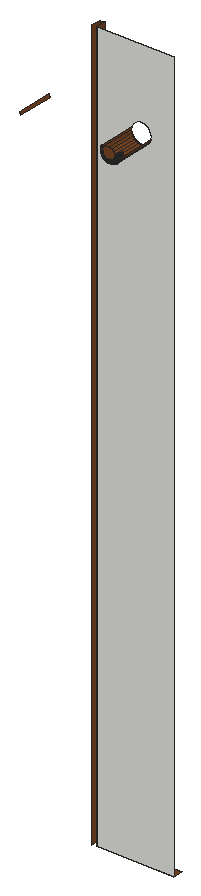
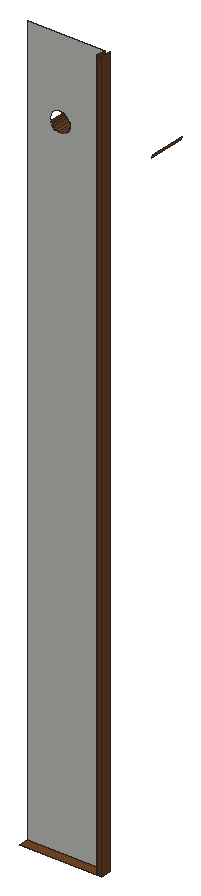
# SketchUp Ruby script. Lengths in inches.
U = 1.inch
M = Sketchup.active_model
def pt(a) = Geom::Point3d.new(a.map { |v| v * U })
def face(e, loops, mat)
  f = e.add_face(loops[0].map { |a| pt(a) })
  loops[1..].each { |l| e.add_face(l.map { |a| pt(a) }).erase! }
  f.material = f.back_material = mat if mat
  f
end
# faces: each face lists its corners as indices into pts; further lists are holes
def faces(e, pts, list, mat = nil) = list.each { |f| face(e, (f[0].is_a?(Array) ? f : [f]).map { |l| l.map { |i| pts[i] } }, mat) }
# xy, xz, yz: faces in a plane at the given z, y or x. An outline is a flat list of corners, or four numbers for a rectangle; further outlines are holes
def ring(l) = l.size == 4 ? [[l[0], l[1]], [l[2], l[1]], [l[2], l[3]], [l[0], l[3]]] : l.each_slice(2).to_a
def flat(e, list, mat, &to3) = list.each { |f| face(e, (f[0].is_a?(Array) ? f : [f]).map { |l| ring(l).map { |u, v| to3.(u, v) } }, mat) }
def xy(e, z, list, mat = nil) = flat(e, list, mat) { |x, y| [x, y, z] }
def xz(e, y, list, mat = nil) = flat(e, list, mat) { |x, z| [x, y, z] }
def yz(e, x, list, mat = nil) = flat(e, list, mat) { |y, z| [x, y, z] }
def lines(e, pts, list) = list.each { |a, b| e.add_line(pt(pts[a]), pt(pts[b])) }
# prism: a flat outline (further loops are holes) pulled along v
def prism(e, loops, v, mat = nil)
  f = face(e, loops, mat); d = Geom::Vector3d.new(v.map { |x| x * U })
  f.pushpull(f.normal.samedirection?(d) ? d.length : -d.length)
end
def box(e, o, s, mat = nil) = prism(e, [[o, [o[0] + s[0], o[1], o[2]], [o[0] + s[0], o[1] + s[1], o[2]], [o[0], o[1] + s[1], o[2]]]], [0, 0, s[2]], mat)
def at(x, y, z, deg = 0) = Geom::Transformation.translation(pt([x, y, z])) * Geom::Transformation.rotation(ORIGIN, Z_AXIS, deg.degrees)
def axes(o, x, y, z) = Geom::Transformation.new([*x, 0, *y, 0, *z, 0, *pt(o).to_a, 1])
def part(name) = M.definitions.add(name)
# library, detail: a bought-in or finely detailed component or shape, given as its bounding box
def library(name, o, s) = part(name).tap { |d| box(d.entities, o, s) }
def detail(e, o, s) = box(e.add_group.entities, o, s)
def put(e, d, t, mat = nil) = e.add_instance(d, t).tap { |i| i.material = mat if mat }
def group(e, t, mat = nil) = e.add_group.tap { |g| g.transformation = t; g.material = mat if mat }.entities
root = M.entities
M.materials.add("[Wood Veneer 01]").color = [120, 70, 37]
xy(root,1.59,[[30.5,2,34.26,2.47]],"[Wood Veneer 01]")
xz(root,0,[[32.68,33.35,32.68,33.36,32.6,33.375,32.59,33.36],[32.68,33.35,32.77,33.36,32.76,33.375,32.68,33.36],[32.59,33.36,32.6,33.375,32.52,33.41,32.51,33.39],[32.68,33.36,32.68,33.38,32.6,33.39,32.6,33.375],[32.68,33.36,32.76,33.375,32.76,33.39,32.68,33.38],
  [32.77,33.36,32.85,33.39,32.84,33.41,32.76,33.375],[32.6,33.375,32.6,33.39,32.53,33.42,32.52,33.41],[32.76,33.375,32.84,33.41,32.83,33.42,32.76,33.39],[32.68,33.38,32.68,33.4,32.61,33.41,32.6,33.39],[32.68,33.38,32.76,33.39,32.75,33.41,32.68,33.4],
  [32.51,33.39,32.52,33.41,32.45,33.46,32.44,33.45],[32.6,33.39,32.61,33.41,32.54,33.4375,32.53,33.42],[32.76,33.39,32.83,33.42,32.82,33.4375,32.75,33.41],[32.85,33.39,32.92,33.45,32.9,33.46,32.84,33.41],[32.68,33.4,32.75,33.41,32.82,33.4375,32.88,33.48,32.93,33.54,32.95,33.61,32.96,33.68,32.95,33.76,32.93,33.83,32.88,33.88,32.82,33.93,32.75,33.96,32.68,33.97,32.61,33.96,32.54,33.93,32.48,33.88,32.43,33.83,32.4,33.76,32.39,33.68,32.4,33.61,32.43,33.54,32.48,33.48,32.54,33.4375,32.61,33.41],
  [32.52,33.41,32.53,33.42,32.47,33.47,32.45,33.46],[32.84,33.41,32.9,33.46,32.89,33.47,32.83,33.42],[32.53,33.42,32.54,33.4375,32.48,33.48,32.47,33.47],[32.83,33.42,32.89,33.47,32.88,33.48,32.82,33.4375],[32.44,33.45,32.45,33.46,32.4,33.52,32.39,33.52],
  [32.92,33.45,32.97,33.52,32.96,33.52,32.9,33.46],[32.45,33.46,32.47,33.47,32.42,33.53,32.4,33.52],[32.9,33.46,32.96,33.52,32.94,33.53,32.89,33.47],[32.47,33.47,32.48,33.48,32.43,33.54,32.42,33.53],[32.89,33.47,32.94,33.53,32.93,33.54,32.88,33.48],
  [32.39,33.52,32.4,33.52,32.37,33.6,32.36,33.6],[32.4,33.52,32.42,33.53,32.39,33.61,32.37,33.6],[32.96,33.52,32.99,33.6,32.97,33.61,32.94,33.53],[32.96,33.52,32.97,33.52,33,33.6,32.99,33.6],[32.42,33.53,32.43,33.54,32.4,33.61,32.39,33.61],
  [32.94,33.53,32.97,33.61,32.95,33.61,32.93,33.54],[32.36,33.6,32.37,33.6,32.36,33.68,32.34,33.68],[32.37,33.6,32.39,33.61,32.38,33.68,32.36,33.68],[32.99,33.6,33,33.68,32.98,33.68,32.97,33.61],[32.99,33.6,33,33.6,33.01,33.68,33,33.68],
  [32.39,33.61,32.4,33.61,32.39,33.68,32.38,33.68],[32.95,33.61,32.97,33.61,32.98,33.68,32.96,33.68],[32.34,33.68,32.36,33.68,32.37,33.77,32.36,33.77],[32.36,33.68,32.38,33.68,32.39,33.76,32.37,33.77],[32.38,33.68,32.39,33.68,32.4,33.76,32.39,33.76],
  [32.96,33.68,32.98,33.68,32.97,33.76,32.95,33.76],[32.98,33.68,33,33.68,32.99,33.77,32.97,33.76],[33,33.68,33.01,33.68,33,33.77,32.99,33.77]],"[Wood Veneer 01]")
xz(root,0.01,[[32.68,33.3,32.68,33.32,32.58,33.33,32.58,33.32],[32.68,33.3,32.78,33.32,32.77,33.33,32.68,33.32],[32.58,33.32,32.58,33.33,32.5,33.37,32.49,33.36],[32.68,33.32,32.68,33.33,32.59,33.34,32.58,33.33],[32.68,33.32,32.77,33.33,32.77,33.34,32.68,33.33],
  [32.78,33.32,32.87,33.36,32.86,33.37,32.77,33.33],[32.58,33.33,32.59,33.34,32.5,33.38,32.5,33.37],[32.77,33.33,32.86,33.37,32.85,33.38,32.77,33.34],[32.49,33.36,32.5,33.37,32.42,33.43,32.41,33.42],[32.87,33.36,32.95,33.42,32.9375,33.43,32.86,33.37],
  [32.5,33.37,32.5,33.38,32.43,33.44,32.42,33.43],[32.86,33.37,32.9375,33.43,32.93,33.44,32.85,33.38],[32.41,33.42,32.42,33.43,32.36,33.5,32.35,33.49],[32.95,33.42,33.01,33.49,33,33.5,32.9375,33.43],[32.42,33.43,32.43,33.44,32.375,33.51,32.36,33.5],
  [32.9375,33.43,33,33.5,32.98,33.51,32.93,33.44],[32.35,33.49,32.36,33.5,32.33,33.59,32.3125,33.59],[33.01,33.49,33.05,33.59,33.03,33.59,33,33.5],[32.36,33.5,32.375,33.51,32.34,33.59,32.33,33.59],[33,33.5,33.03,33.59,33.02,33.59,32.98,33.51],
  [32.3125,33.59,32.33,33.59,32.3125,33.68,32.3,33.68],[32.33,33.59,32.34,33.59,32.33,33.68,32.3125,33.68],[33.02,33.59,33.03,33.59,33.04,33.68,33.03,33.68],[33.03,33.59,33.05,33.59,33.06,33.68,33.04,33.68],[32.3,33.68,32.3125,33.68,32.33,33.78,32.3125,33.78],
  [32.3125,33.68,32.33,33.68,32.34,33.77,32.33,33.78],[33.03,33.68,33.04,33.68,33.03,33.78,33.02,33.77],[33.04,33.68,33.06,33.68,33.05,33.78,33.03,33.78]],"[Wood Veneer 01]")
xz(root,0.02,[[32.68,33.28,32.68,33.29,32.58,33.3,32.57,33.29],[32.68,33.28,32.78,33.29,32.78,33.3,32.68,33.29],[32.57,33.29,32.58,33.3,32.48,33.34,32.48,33.33],[32.78,33.29,32.88,33.33,32.875,33.34,32.78,33.3],[32.48,33.33,32.48,33.34,32.4,33.41,32.39,33.4],
  [32.88,33.33,32.97,33.4,32.96,33.41,32.875,33.34],[32.39,33.4,32.4,33.41,32.34,33.49,32.33,33.48],[32.97,33.4,33.03,33.48,33.02,33.49,32.96,33.41],[32.33,33.48,32.34,33.49,32.3,33.58,32.29,33.58],[33.03,33.48,33.07,33.58,33.06,33.58,33.02,33.49],
  [32.29,33.58,32.3,33.58,32.29,33.68,32.28,33.68],[33.06,33.58,33.07,33.58,33.08,33.68,33.07,33.68],[32.28,33.68,32.29,33.68,32.3,33.78,32.29,33.79],[33.07,33.68,33.08,33.68,33.07,33.79,33.06,33.78]],"[Wood Veneer 01]")
xz(root,0.04,[[32.68,33.25,32.68,33.26,32.57,33.27,32.57,33.26],[32.68,33.25,32.79,33.26,32.79,33.27,32.68,33.26],[32.57,33.26,32.57,33.27,32.47,33.3125,32.46,33.31],[32.79,33.26,32.9,33.31,32.89,33.3125,32.79,33.27],[32.46,33.31,32.47,33.3125,32.38,33.38,32.37,33.375],
  [32.9,33.31,32.99,33.375,32.98,33.38,32.89,33.3125],[32.37,33.375,32.38,33.38,32.31,33.47,32.3,33.46],[32.99,33.375,33.06,33.46,33.05,33.47,32.98,33.38],[32.3,33.46,32.31,33.47,32.27,33.57,32.26,33.57],[33.06,33.46,33.1,33.57,33.09,33.57,33.05,33.47],
  [32.26,33.57,32.27,33.57,32.25,33.68,32.24,33.68],[33.09,33.57,33.1,33.57,33.12,33.68,33.11,33.68],[32.24,33.68,32.25,33.68,32.27,33.79,32.26,33.8],[33.11,33.68,33.12,33.68,33.1,33.8,33.09,33.79]],"[Wood Veneer 01]")
xz(root,2,[[[30.5,1.59,34.26,37.59],[32.68,33.18,32.55,33.2,32.43,33.25,32.33,33.33,32.25,33.43,32.2,33.55,32.18,33.68,32.2,33.8125,32.25,33.93,32.33,34.04,32.43,34.12,32.55,34.17,32.68,34.18,32.81,34.17,32.93,34.12,33.03,34.04,33.11,33.93,33.16,33.8125,33.18,33.68,33.16,33.55,33.11,33.43,33.03,33.33,32.93,33.25,32.81,33.2]]])
xz(root,2.47,[[30.26,1.59,30.5,37.59]],"[Wood Veneer 01]")
yz(root,30.26,[[2,1.59,2.47,37.59]],"[Wood Veneer 01]")
yz(root,30.5,[[2,1.59,2.47,37.59]],"[Wood Veneer 01]")
p = [[32.5625,0.05,33.25],[32.68,0.05,33.24],[32.68,0.04,33.25],[32.57,0.04,33.26],[32.79,0.04,33.26],[32.79,0.05,33.25],
  [32.55,0.15,33.21],[32.43,0.15,33.26],[32.43,0.16,33.25],[32.55,0.16,33.2],[32.55,0.13,33.21],[32.43,0.13,33.26],
  [32.55,0.12,33.21],[32.4375,0.12,33.26],[32.55,0.11,33.22],[32.4375,0.11,33.27],[32.56,0.09,33.22],[32.44,0.09,33.27],
  [32.56,0.08,33.23],[32.44,0.08,33.28],[32.56,0.07,33.24],[32.45,0.07,33.28],[32.5625,0.0625,33.24],[32.45,0.0625,33.29],
  [32.46,0.05,33.3],[32.68,0.16,33.1875],[32.68,0.15,33.1875],[32.68,0.13,33.19],[32.68,0.12,33.2],[32.68,0.11,33.2],
  [32.68,0.09,33.21],[32.68,0.08,33.21],[32.68,0.07,33.22],[32.68,0.0625,33.23],[32.8,0.0625,33.24],[32.8,0.07,33.24],
  [32.8,0.08,33.23],[32.8,0.09,33.22],[32.8,0.11,33.22],[32.81,0.12,33.21],[32.81,0.13,33.21],[32.81,0.15,33.21],
  [32.81,0.16,33.2],[32.91,0.0625,33.29],[32.9,0.05,33.3],[32.91,0.07,33.28],[32.91,0.08,33.28],[32.92,0.09,33.27],
  [32.92,0.11,33.27],[32.92,0.12,33.26],[32.92,0.13,33.26],[32.93,0.15,33.26],[32.93,0.16,33.25],[32.43,2,33.25],
  [32.55,2,33.2],[32.55,0.21,33.2],[32.43,0.21,33.25],[32.55,0.2,33.2],[32.43,0.2,33.25],[32.55,0.18,33.2],
  [32.43,0.18,33.25],[32.68,2,33.18],[32.68,0.21,33.18],[32.68,0.2,33.18],[32.68,0.18,33.18],[32.81,0.18,33.2],
  [32.81,0.2,33.2],[32.81,0.21,33.2],[32.81,2,33.2],[32.93,0.18,33.25],[32.93,0.2,33.25],[32.93,0.21,33.25],
  [32.93,2,33.25],[32.36,0.05,33.37],[32.46,0.04,33.31],[32.37,0.04,33.375],[32.38,0.04,33.38],[32.47,0.04,33.3125],
  [32.47,0.03,33.32],[32.39,0.03,33.39],[32.48,0.02,33.33],[32.39,0.02,33.4],[32.4,0.02,33.41],[32.48,0.02,33.34],
  [32.49,0.01,33.36],[32.41,0.01,33.42],[32.57,0.03,33.28],[32.57,0.04,33.27],[32.57,0.02,33.29],[32.58,0.01,33.32],
  [32.58,0.02,33.3],[32.59,0,33.36],[32.51,0,33.39],[32.5,0.01,33.38],[32.59,0.01,33.34],[32.68,0.04,33.26],
  [32.68,0.03,33.27],[32.68,0.02,33.28],[32.68,0.02,33.29],[32.68,0.01,33.3],[32.68,0.01,33.33],[32.68,0,33.35],
  [32.77,0,33.36],[32.77,0.01,33.34],[32.78,0.01,33.32],[32.78,0.02,33.3],[32.78,0.02,33.29],[32.79,0.03,33.28],
  [32.79,0.04,33.27],[32.85,0.01,33.38],[32.85,0,33.39],[32.875,0.02,33.34],[32.87,0.01,33.36],[32.89,0.03,33.32],
  [32.88,0.02,33.33],[32.89,0.04,33.3125],[32.9,0.04,33.31],[32.96,0.02,33.41],[32.95,0.01,33.42],[32.97,0.03,33.39],
  [32.97,0.02,33.4],[32.98,0.04,33.38],[32.99,0.05,33.37],[32.99,0.04,33.375],[32.33,0.15,33.33],[32.25,0.15,33.4375],
  [32.25,0.16,33.43],[32.33,0.16,33.33],[32.33,0.13,33.34],[32.25,0.13,33.4375],[32.34,0.12,33.34],[32.26,0.12,33.44],
  [32.34,0.11,33.34],[32.26,0.11,33.44],[32.34,0.09,33.35],[32.27,0.09,33.45],[32.35,0.08,33.35],[32.27,0.08,33.45],
  [32.35,0.07,33.36],[32.36,0.0625,33.36],[33,0.0625,33.36],[33.01,0.07,33.36],[33.01,0.08,33.35],[33.02,0.09,33.35],
  [33.02,0.11,33.34],[33.02,0.12,33.34],[33.03,0.13,33.34],[33.03,0.15,33.33],[33.03,0.16,33.33],[33.09,0.09,33.45],
  [33.09,0.08,33.45],[33.1,0.11,33.44],[33.1,0.12,33.44],[33.1,0.13,33.4375],[33.11,0.15,33.4375],[33.11,0.16,33.43],
  [32.25,2,33.43],[32.33,2,33.33],[32.33,0.21,33.33],[32.25,0.21,33.43],[32.33,0.2,33.33],[32.25,0.2,33.43],
  [32.33,0.18,33.33],[32.25,0.18,33.43],[33.03,0.18,33.33],[33.03,0.2,33.33],[33.03,0.21,33.33],[33.03,2,33.33],
  [33.11,0.18,33.43],[33.11,0.2,33.43],[33.11,0.21,33.43],[33.11,2,33.43],[32.3,0.04,33.46],[32.29,0.05,33.46],
  [32.32,0.03,33.48],[32.31,0.04,33.47],[32.33,0.02,33.48],[32.35,0.01,33.49],[32.34,0.02,33.49],[32.44,0,33.45],
  [32.39,0,33.52],[32.375,0.01,33.51],[32.43,0.01,33.44],[32.93,0.01,33.44],[32.92,0,33.45],[32.98,0.01,33.51],
  [32.97,0,33.52],[33.02,0.02,33.49],[33.01,0.01,33.49],[33.04,0.03,33.48],[33.03,0.02,33.48],[33.05,0.04,33.47],
  [33.07,0.05,33.46],[33.06,0.04,33.46],[32.2,0.16,33.55],[32.2,0.15,33.56],[32.21,0.13,33.56],[32.21,0.12,33.56],
  [32.21,0.11,33.56],[32.22,0.09,33.56],[32.23,0.08,33.5625],[32.28,0.07,33.45],[32.23,0.07,33.5625],[32.29,0.0625,33.46],
  [33.07,0.0625,33.46],[33.08,0.07,33.45],[33.125,0.07,33.5625],[33.13,0.08,33.5625],[33.14,0.09,33.56],[33.14,0.11,33.56],
  [33.15,0.12,33.56],[33.15,0.13,33.56],[33.16,0.15,33.56],[33.16,0.16,33.55],[32.2,2,33.55],[32.2,0.21,33.55],
  [32.2,0.2,33.55],[32.2,0.18,33.55],[33.16,0.18,33.55],[33.16,0.2,33.55],[33.16,0.21,33.55],[33.16,2,33.55],
  [32.25,0.05,33.57],[32.26,0.04,33.57],[32.27,0.04,33.57],[32.28,0.03,33.58],[32.29,0.02,33.58],[32.3,0.02,33.58],
  [32.3125,0.01,33.59],[32.34,0.01,33.59],[32.36,0,33.6],[33,0,33.6],[33.02,0.01,33.59],[33.05,0.01,33.59],
  [33.06,0.02,33.58],[33.07,0.02,33.58],[33.08,0.03,33.58],[33.09,0.04,33.57],[33.1,0.04,33.57],[33.11,0.05,33.57],
  [32.24,0.0625,33.57],[33.12,0.0625,33.57],[32.23,0.05,33.68],[32.24,0.04,33.68],[32.25,0.04,33.68],[32.26,0.03,33.68],
  [32.28,0.02,33.68],[32.29,0.02,33.68],[32.3,0.01,33.68],[32.33,0.01,33.68],[32.34,0,33.68],[33.01,0,33.68],
  [33.03,0.01,33.68],[33.06,0.01,33.68],[33.07,0.02,33.68],[33.08,0.02,33.68],[33.1,0.03,33.68],[33.11,0.04,33.68],
  [33.12,0.04,33.68],[33.125,0.05,33.68],[32.18,0.16,33.68],[32.19,0.15,33.68],[32.1875,0.13,33.68],[32.19,0.12,33.68],
  [32.2,0.11,33.68],[32.2,0.09,33.68],[32.21,0.08,33.68],[32.22,0.07,33.68],[32.22,0.0625,33.68],[33.13,0.0625,33.68],
  [33.14,0.07,33.68],[33.15,0.08,33.68],[33.16,0.09,33.68],[33.16,0.11,33.68],[33.17,0.12,33.68],[33.17,0.13,33.68],
  [33.17,0.15,33.68],[33.18,0.16,33.68],[32.18,2,33.68],[32.18,0.21,33.68],[32.18,0.2,33.68],[32.18,0.18,33.68],
  [33.18,0.18,33.68],[33.18,0.2,33.68],[33.18,0.21,33.68],[32.25,0.05,33.8],[32.26,0.04,33.8],[32.27,0.04,33.79],
  [32.28,0.03,33.79],[32.29,0.02,33.79],[32.3,0.02,33.78],[32.3125,0.01,33.78],[32.34,0.01,33.77],[32.36,0,33.77],
  [33.02,0.01,33.77],[33,0,33.77],[33.06,0.02,33.78],[33.05,0.01,33.78],[33.08,0.03,33.79],[33.07,0.02,33.79],
  [33.09,0.04,33.79],[33.11,0.05,33.8],[33.1,0.04,33.8],[32.2,0.16,33.8125],[32.2,0.15,33.8125],[32.21,0.13,33.81],
  [32.21,0.12,33.81],[32.21,0.11,33.81],[32.22,0.09,33.81],[32.23,0.08,33.8],[32.23,0.07,33.8],[32.24,0.0625,33.8],
  [33.12,0.0625,33.8],[33.125,0.07,33.8],[33.13,0.08,33.8],[33.14,0.09,33.81],[33.14,0.11,33.81],[33.15,0.12,33.81],
  [33.15,0.13,33.81],[33.16,0.15,33.8125],[33.16,0.16,33.8125],[28.18,2,33.68],[28.16,2,33.8125],[28.16,0.22,33.8125],
  [28.18,0.22,33.68],[32.2,2,33.8125],[32.2,0.21,33.8125],[32.2,0.2,33.8125],[32.2,0.18,33.8125],[33.16,0.18,33.8125],
  [33.16,0.2,33.8125],[33.16,0.21,33.8125]]
faces(root,p,[[0,1,2,3],[4,2,1,5],[6,7,8,9],[10,11,7,6],[12,13,11,10],[14,15,13,12],[16,17,15,14],[18,19,17,16],
  [20,21,19,18],[22,23,21,20],[0,24,23,22],[9,25,26,6],[6,26,27,10],[10,27,28,12],[12,28,29,14],[14,29,30,16],
  [16,30,31,18],[18,31,32,20],[20,32,33,22],[22,33,1,0],[5,1,33,34],[34,33,32,35],[35,32,31,36],[36,31,30,37],
  [37,30,29,38],[38,29,28,39],[39,28,27,40],[40,27,26,41],[41,26,25,42],[34,43,44,5],[35,45,43,34],[36,46,45,35],
  [37,47,46,36],[38,48,47,37],[39,49,48,38],[40,50,49,39],[41,51,50,40],[42,52,51,41],[53,54,55,56],[57,58,56,55],
  [59,60,58,57],[9,8,60,59],[54,61,62,55],[55,62,63,57],[57,63,64,59],[59,64,25,9],[42,25,64,65],[65,64,63,66],
  [66,63,62,67],[61,68,67,62],[65,69,52,42],[66,70,69,65],[67,71,70,66],[68,72,71,67],[73,24,74,75],[76,77,78,79],
  [79,78,80,81],[82,83,84,85],[3,74,24,0],[86,78,77,87],[88,80,78,86],[89,84,83,90],[91,92,93,94],[87,95,96,86],
  [86,96,97,88],[90,98,99,89],[94,100,101,91],[102,101,100,103],[104,99,98,105],[106,97,96,107],[107,96,95,108],[103,109,110,102],
  [105,111,112,104],[107,113,114,106],[108,115,113,107],[5,44,116,4],[111,117,118,112],[113,119,120,114],[115,121,119,113],[44,122,123,116],
  [124,125,126,127],[128,129,125,124],[130,131,129,128],[132,133,131,130],[134,135,133,132],[136,137,135,134],[127,8,7,124],[124,7,11,128],
  [128,11,13,130],[130,13,15,132],[132,15,17,134],[134,17,19,136],[136,19,21,138],[138,21,23,139],[139,23,24,73],[43,140,122,44],
  [45,141,140,43],[46,142,141,45],[47,143,142,46],[48,144,143,47],[49,145,144,48],[50,146,145,49],[51,147,146,50],[52,148,147,51],
  [143,149,150,142],[144,151,149,143],[145,152,151,144],[146,153,152,145],[147,154,153,146],[148,155,154,147],[156,157,158,159],[160,161,159,158],
  [162,163,161,160],[127,126,163,162],[157,53,56,158],[158,56,58,160],[160,58,60,162],[162,60,8,127],[69,164,148,52],[70,165,164,69],
  [71,166,165,70],[72,167,166,71],[164,168,155,148],[165,169,168,164],[166,170,169,165],[167,171,170,166],[75,172,173,73],[79,174,175,76],
  [81,176,174,79],[85,177,178,82],[179,180,181,182],[182,93,92,179],[109,183,184,110],[183,185,186,184],[117,187,188,118],[119,189,190,120],
  [121,191,189,119],[122,192,193,123],[194,126,125,195],[195,125,129,196],[196,129,131,197],[197,131,133,198],[198,133,135,199],[199,135,137,200],
  [200,137,201,202],[138,201,137,136],[139,203,201,138],[73,173,203,139],[140,204,192,122],[141,205,204,140],[142,150,205,141],[206,205,150,207],
  [207,150,149,208],[208,149,151,209],[209,151,152,210],[210,152,153,211],[211,153,154,212],[212,154,155,213],[214,156,159,215],[215,159,161,216],
  [216,161,163,217],[217,163,126,194],[213,155,168,218],[218,168,169,219],[219,169,170,220],[171,221,220,170],[222,173,172,223],[224,175,174,225],
  [225,174,176,226],[227,178,177,228],[229,181,180,230],[231,186,185,232],[233,188,187,234],[235,190,189,236],[236,189,191,237],[238,193,192,239],
  [202,201,203,240],[240,203,173,222],[239,192,204,241],[241,204,205,206],[242,222,223,243],[244,224,225,245],[245,225,226,246],[247,227,228,248],
  [249,229,230,250],[251,231,232,252],[253,233,234,254],[255,235,236,256],[256,236,237,257],[258,238,239,259],[260,194,195,261],[261,195,196,262],
  [262,196,197,263],[263,197,198,264],[264,198,199,265],[265,199,200,266],[266,200,202,267],[267,202,240,268],[268,240,222,242],[259,239,241,269],
  [269,241,206,270],[270,206,207,271],[271,207,208,272],[272,208,209,273],[273,209,210,274],[274,210,211,275],[275,211,212,276],[276,212,213,277],
  [278,214,215,279],[279,215,216,280],[280,216,217,281],[281,217,194,260],[277,213,218,282],[282,218,219,283],[283,219,220,284],[285,242,243,286],
  [287,244,245,288],[288,245,246,289],[290,247,248,291],[292,249,250,293],[252,294,295,251],[254,296,297,253],[256,298,299,255],[257,300,298,256],
  [259,301,302,258],[303,260,261,304],[304,261,262,305],[305,262,263,306],[306,263,264,307],[307,264,265,308],[308,265,266,309],[309,266,267,310],
  [310,267,268,311],[311,268,242,285],[269,312,301,259],[270,313,312,269],[271,314,313,270],[272,315,314,271],[273,316,315,272],[274,317,316,273],
  [275,318,317,274],[276,319,318,275],[277,320,319,276],[321,322,323,324],[325,278,279,326],[326,279,280,327],[327,280,281,328],[328,281,260,303],
  [282,329,320,277],[283,330,329,282],[284,331,330,283]],"[Wood Veneer 01]")
